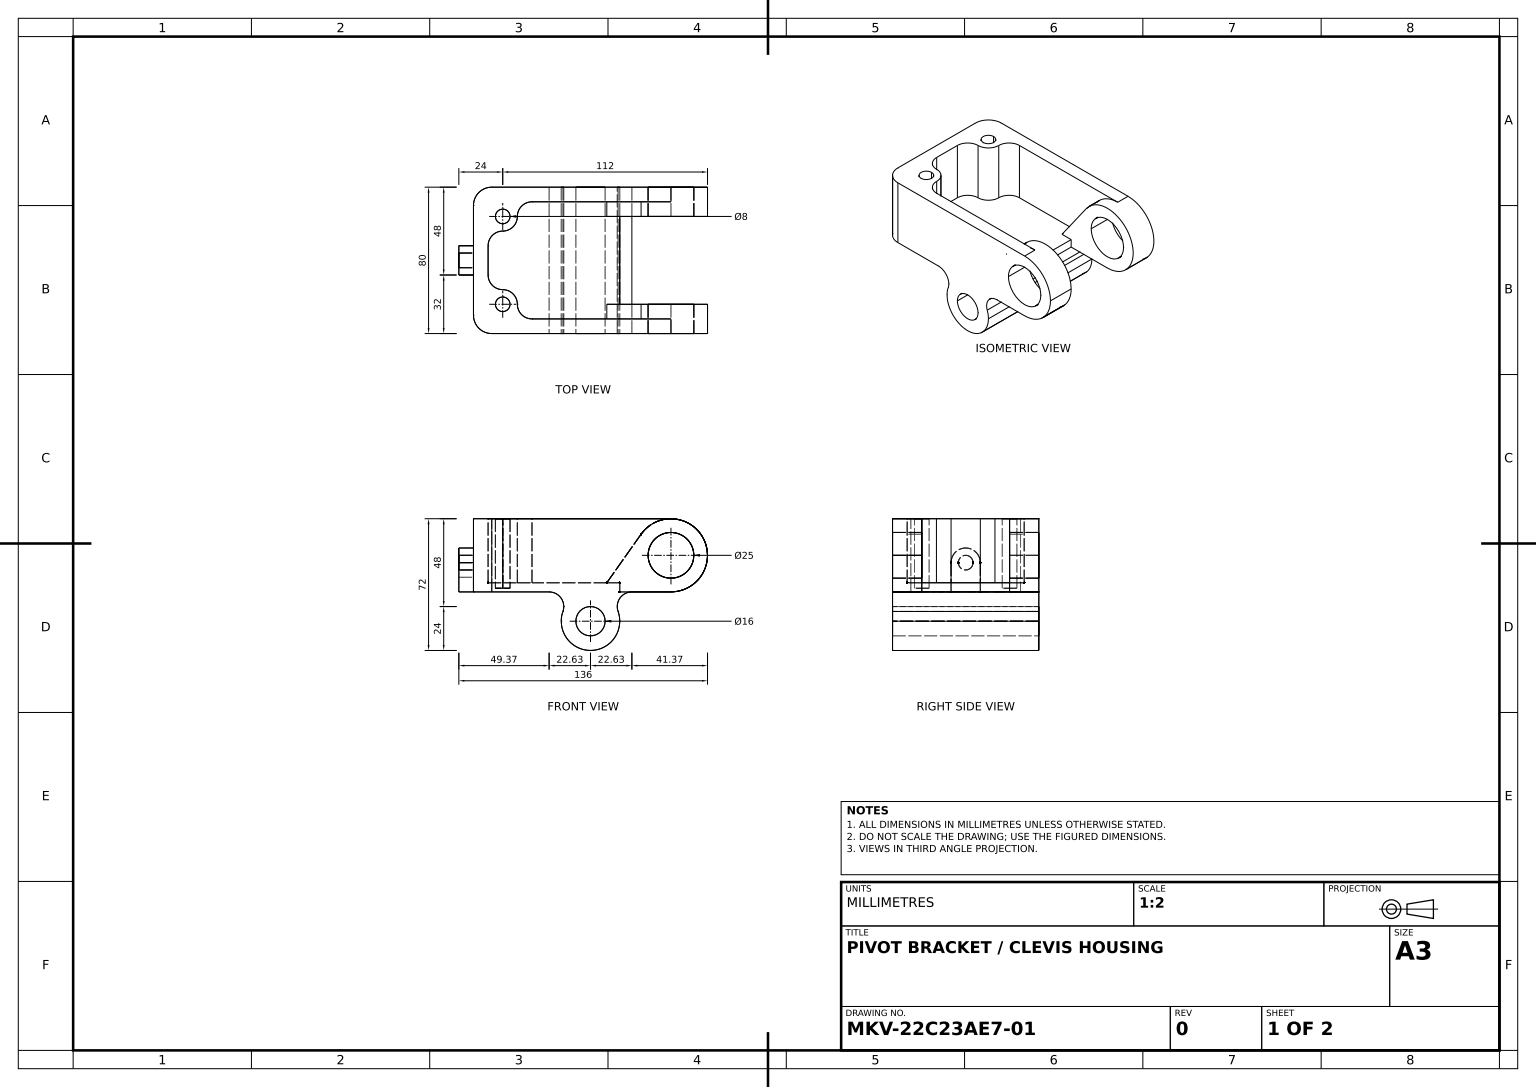
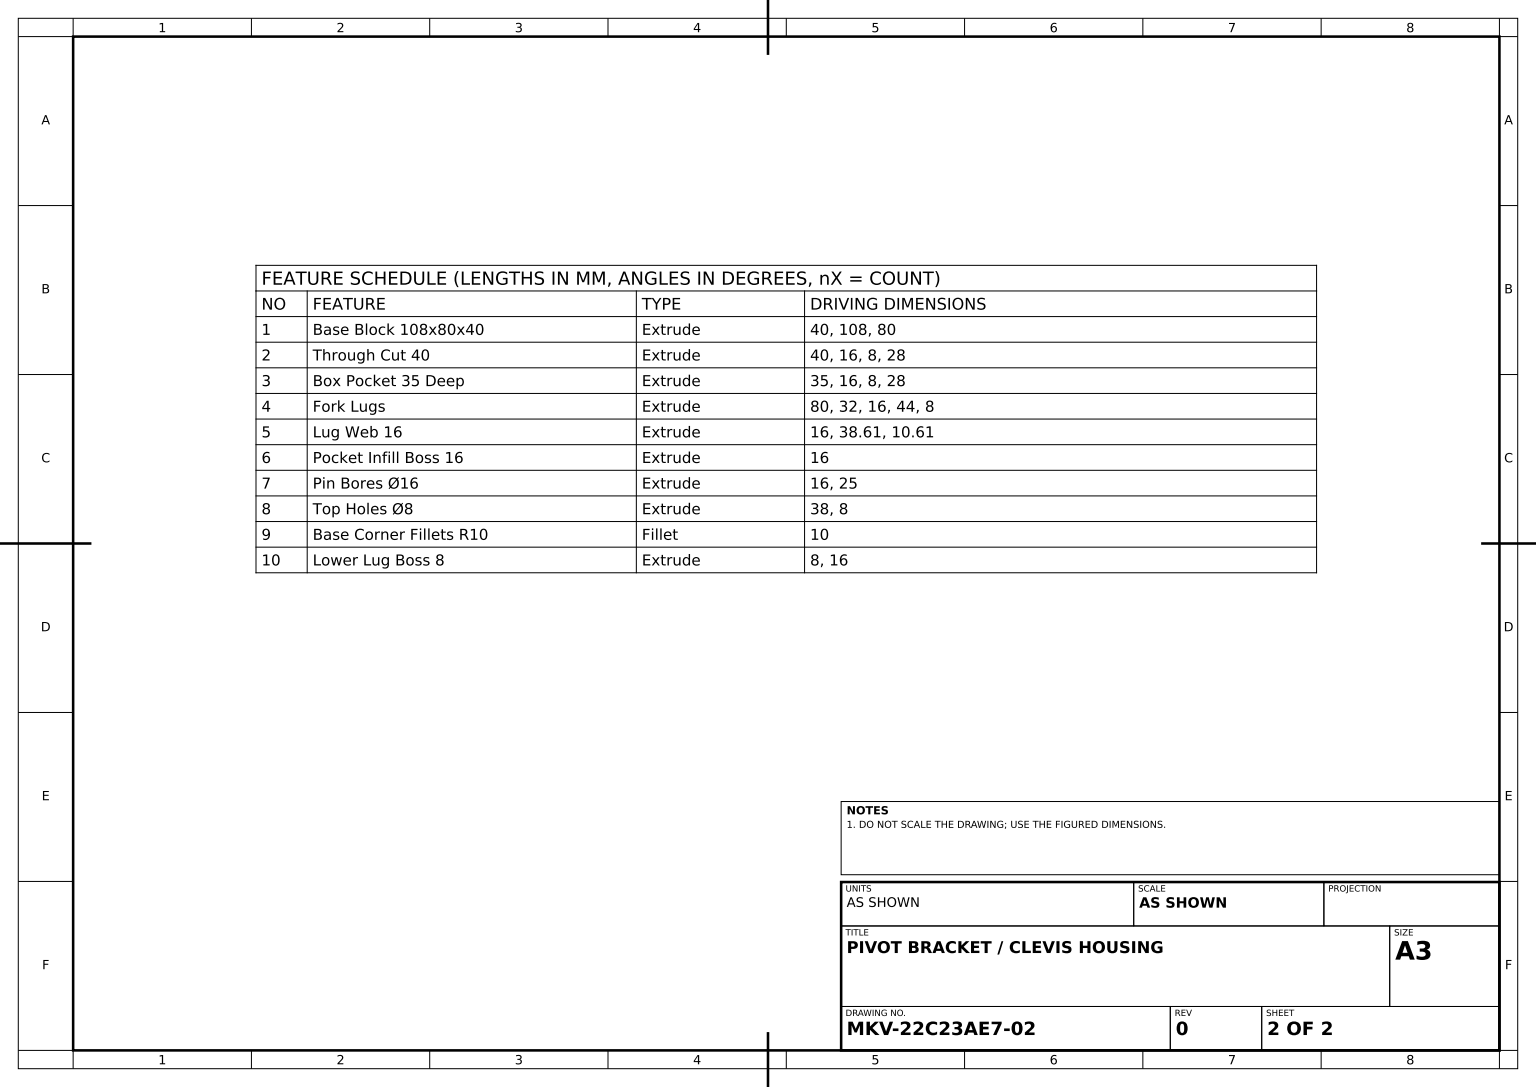
solid
v1 (-38,2,-20)
v2 (-38,40,-20)
e1 v1 v2 LINE
v3 (-38,2,-28)
e2 v3 v1 CIRCLE(AX(P(-38,2,-24),D(0,1,0),D(0,0,1)),4)
v4 (-38,40,-28)
e3 v3 v4 LINE
e4 v4 v2 CIRCLE(AX(P(-38,40,-24),D(0,1,0),D(0,0,1)),4)
face CYL(AX(P(-38,2,-24),D(0,1,0),D(0,0,1)),4) rev [-e1 -e2 e3 e4]
v5 (-38,2,28)
v6 (-38,2,20)
e5 v5 v6 CIRCLE(AX(P(-38,2,24),D(0,1,0),D(0,0,1)),4)
e6 v6 v5 CIRCLE(AX(P(-38,2,24),D(0,1,0),D(0,0,1)),4)
face PLANE(AX(P(-38,2,24),D(0,1,0),D(0,0,1))) [e5 e6]
v7 (-5.084945,-10.666667,-40)
v8 (-5.084945,-10.666667,40)
e7 v7 v8 LINE
v9 (-6,-16,-40)
e8 v7 v9 CIRCLE(AX(P(10,-16,-40),D(0,0,1),D(1,0,0)),16)
v10 (-6,-16,40)
e9 v9 v10 LINE
e10 v8 v10 CIRCLE(AX(P(10,-16,40),D(0,0,1),D(1,0,0)),16)
face CYL(AX(P(10,-16,-40),D(0,0,1),D(1,0,0)),16) [-e7 e8 e9 -e10]
v11 (74,20,24)
v12 (74,20,40)
e11 v11 v12 LINE
v13 (54,0,40)
e12 v13 v12 CIRCLE(AX(P(54,20,40),D(0,0,1),D(1,0,0)),20)
v14 (54,0,24)
e13 v13 v14 LINE
e14 v14 v11 CIRCLE(AX(P(54,20,24),D(0,0,1),D(1,0,0)),20)
face CYL(AX(P(54,20,24),D(0,0,1),D(1,0,0)),20) [e11 -e12 e13 e14]
v15 (66.5,20,24)
v16 (66.5,20,40)
e15 v15 v16 LINE
v17 (41.5,20,24)
e16 v15 v17 CIRCLE(AX(P(54,20,24),D(0,0,-1),D(-1,0,0)),12.5)
v18 (41.5,20,40)
e17 v17 v18 LINE
e18 v18 v16 CIRCLE(AX(P(54,20,40),D(0,0,1),D(1,0,0)),12.5)
face CYL(AX(P(54,20,-40),D(0,0,1),D(1,0,0)),12.5) rev [-e15 e16 e17 e18]
v19 (-30,5,24)
v20 (-38,5,16)
e19 v19 v20 CIRCLE(AX(P(-38,5,24),D(0,1,0),D(0,0,1)),8)
v21 (-38,40,16)
e20 v20 v21 LINE
v22 (-30,40,24)
e21 v22 v21 CIRCLE(AX(P(-38,40,24),D(0,1,0),D(0,0,1)),8)
e22 v19 v22 LINE
face CYL(AX(P(-38,5,24),D(0,1,0),D(0,0,1)),8) [e19 e20 -e21 -e22]
e23 v2 v4 CIRCLE(AX(P(-38,40,-24),D(0,1,0),D(0,0,1)),4)
e24 v1 v3 CIRCLE(AX(P(-38,2,-24),D(0,1,0),D(0,0,1)),4)
face CYL(AX(P(-38,2,-24),D(0,1,0),D(0,0,1)),4) rev [e23 -e3 -e24 e1]
v23 (-54,16,4)
v24 (-54,16,-4)
e25 v23 v24 CIRCLE(AX(P(-54,16,0),D(-1,0,0),D(0,0,1)),4)
v25 (-62,16,4)
e26 v25 v23 LINE
v26 (-62,16,-4)
e27 v25 v26 CIRCLE(AX(P(-62,16,0),D(-1,0,0),D(0,0,1)),4)
e28 v26 v24 LINE
face CYL(AX(P(-62,16,0),D(1,0,0),D(0,0,-1)),4) rev [-e25 -e26 e27 e28]
v27 (-22,5,-32)
v28 (-22,40,-32)
e29 v27 v28 LINE
v29 (-30,40,-24)
e30 v29 v28 CIRCLE(AX(P(-22,40,-24),D(0,-1,0),D(0,0,1)),8)
v30 (-30,5,-24)
e31 v30 v29 LINE
e32 v30 v27 CIRCLE(AX(P(-22,5,-24),D(0,-1,0),D(0,0,1)),8)
face CYL(AX(P(-22,5,-24),D(0,1,0),D(0,0,1)),8) rev [e29 -e30 -e31 e32]
e33 v24 v23 CIRCLE(AX(P(-54,16,0),D(-1,0,0),D(0,0,1)),4)
face PLANE(AX(P(-54,40,40),D(1,0,0),D(0,0,-1))) rev [e33 e25]
v31 (-44,0,40)
v32 (-54,0,30)
e34 v31 v32 CIRCLE(AX(P(-44,0,30),D(0,-1,0),D(0,0,-1)),10)
v33 (-54,0,8)
e35 v33 v32 LINE
v34 (-62,0,8)
e36 v34 v33 LINE
v35 (-62,0,-8)
e37 v35 v34 LINE
v36 (-54,0,-8)
e38 v35 v36 LINE
v37 (-54,0,-30)
e39 v37 v36 LINE
v38 (-44,0,-40)
e40 v37 v38 CIRCLE(AX(P(-44,0,-30),D(0,-1,0),D(0,0,-1)),10)
v39 (-12.627417,0,-40)
e41 v39 v38 LINE
v40 (-12.627417,0,40)
e42 v39 v40 LINE
e43 v31 v40 LINE
face PLANE(AX(P(0,0,0),D(0,-1,0),D(0,0,-1))) [e34 -e35 -e36 -e37 e38 -e39 e40 -e41 e42 -e43]
v41 (66.5,20,-40)
v42 (66.5,20,-24)
e44 v41 v42 LINE
v43 (41.5,20,-24)
e45 v43 v42 CIRCLE(AX(P(54,20,-24),D(0,0,-1),D(-1,0,0)),12.5)
v44 (41.5,20,-40)
e46 v44 v43 LINE
e47 v41 v44 CIRCLE(AX(P(54,20,-40),D(0,0,1),D(1,0,0)),12.5)
face CYL(AX(P(54,20,-40),D(0,0,1),D(1,0,0)),12.5) rev [e44 -e45 -e46 -e47]
v45 (-62,16,-8)
v46 (-54,16,-8)
e48 v45 v46 LINE
v47 (-62,16,8)
e49 v47 v45 CIRCLE(AX(P(-62,16,0),D(-1,0,0),D(0,0,1)),8)
v48 (-54,16,8)
e50 v47 v48 LINE
e51 v48 v46 CIRCLE(AX(P(-54,16,0),D(-1,0,0),D(0,0,1)),8)
face CYL(AX(P(-62,16,0),D(1,0,0),D(0,0,-1)),8) [-e48 -e49 e50 e51]
v49 (2,-16,-40)
v50 (18,-16,-40)
e52 v49 v50 CIRCLE(AX(P(10,-16,-40),D(0,0,1),D(1,0,0)),8)
e53 v50 v49 CIRCLE(AX(P(10,-16,-40),D(0,0,1),D(1,0,0)),8)
e54 v44 v41 CIRCLE(AX(P(54,20,-40),D(0,0,1),D(1,0,0)),12.5)
v51 (-4.627417,-8,-40)
e55 v51 v7 CIRCLE(AX(P(-12.627417,-8,-40),D(0,0,-1),D(-1,0,0)),8)
e56 v39 v51 CIRCLE(AX(P(-12.627417,-8,-40),D(0,0,-1),D(-1,0,0)),8)
v52 (-44,40,-40)
e57 v38 v52 LINE
v53 (54,40,-40)
e58 v53 v52 LINE
v54 (54,0,-40)
e59 v53 v54 CIRCLE(AX(P(54,20,-40),D(0,0,-1),D(-1,0,0)),20)
v55 (32.627417,0,-40)
e60 v54 v55 LINE
v56 (25.084945,-10.666667,-40)
e61 v56 v55 CIRCLE(AX(P(32.627417,-8,-40),D(0,0,-1),D(-1,0,0)),8)
v57 (26,-16,-40)
e62 v57 v56 CIRCLE(AX(P(10,-16,-40),D(0,0,1),D(1,0,0)),16)
e63 v9 v57 CIRCLE(AX(P(10,-16,-40),D(0,0,1),D(1,0,0)),16)
face PLANE(AX(P(-54,40,-40),D(0,0,1),D(1,0,0))) rev [e52 e53] [e54 e47] [-e8 -e55 -e56 e41 e57 -e58 e59 e60 -e61 -e62 -e63]
v58 (26,5,24)
v59 (18.921249,5,24)
e64 v58 v59 LINE
v60 (37.663471,31.537669,24)
e65 v60 v59 LINE
e66 v11 v60 CIRCLE(AX(P(54,20,24),D(0,0,1),D(1,0,0)),20)
v61 (32.627417,0,24)
e67 v61 v14 LINE
v62 (26,0,24)
e68 v61 v62 LINE
e69 v58 v62 LINE
e70 v17 v15 CIRCLE(AX(P(54,20,24),D(0,0,-1),D(-1,0,0)),12.5)
face PLANE(AX(P(32.627417,-8,24),D(0,0,-1),D(-1,0,0))) [e64 -e65 -e66 -e14 -e67 e68 -e69] [-e70 -e16]
v63 (32.627417,0,-24)
e71 v55 v63 LINE
e72 v63 v61 LINE
v64 (32.627417,0,40)
e73 v61 v64 LINE
v65 (25.084945,-10.666667,40)
e74 v65 v64 CIRCLE(AX(P(32.627417,-8,40),D(0,0,-1),D(-1,0,0)),8)
e75 v56 v65 LINE
face CYL(AX(P(32.627417,-8,-40),D(0,0,1),D(1,0,0)),8) rev [e61 e71 e72 e73 -e74 -e75]
v66 (18,-16,40)
e76 v50 v66 LINE
v67 (2,-16,40)
e77 v66 v67 CIRCLE(AX(P(10,-16,40),D(0,0,1),D(1,0,0)),8)
e78 v49 v67 LINE
face CYL(AX(P(10,-16,-40),D(0,0,1),D(1,0,0)),8) rev [e76 e77 -e78 -e53]
v68 (-54,40,-30)
e79 v52 v68 CIRCLE(AX(P(-44,40,-30),D(0,1,0),D(0,0,-1)),10)
v69 (-54,40,30)
e80 v68 v69 LINE
v70 (-44,40,40)
e81 v69 v70 CIRCLE(AX(P(-44,40,30),D(0,1,0),D(0,0,-1)),10)
v71 (54,40,40)
e82 v70 v71 LINE
v72 (54,40,32)
e83 v71 v72 LINE
v73 (-22,40,32)
e84 v72 v73 LINE
e85 v22 v73 CIRCLE(AX(P(-22,40,24),D(0,1,0),D(0,0,1)),8)
v74 (-46,40,8)
e86 v74 v21 CIRCLE(AX(P(-38,40,8),D(0,1,0),D(0,0,1)),8)
v75 (-46,40,-8)
e87 v74 v75 LINE
v76 (-38,40,-16)
e88 v75 v76 CIRCLE(AX(P(-38,40,-8),D(0,-1,0),D(0,0,1)),8)
e89 v76 v29 CIRCLE(AX(P(-38,40,-24),D(0,1,0),D(0,0,1)),8)
v77 (54,40,-32)
e90 v77 v28 LINE
e91 v77 v53 LINE
v78 (-38,40,20)
v79 (-38,40,28)
e92 v78 v79 CIRCLE(AX(P(-38,40,24),D(0,1,0),D(0,0,1)),4)
e93 v79 v78 CIRCLE(AX(P(-38,40,24),D(0,1,0),D(0,0,1)),4)
face PLANE(AX(P(0,40,0),D(0,-1,0),D(0,0,-1))) rev [e79 e80 e81 e82 e83 e84 -e85 e21 -e86 e87 e88 e89 e30 -e90 e91 e58] [-e4 -e23] [-e92 -e93]
e94 v64 v13 LINE
face PLANE(AX(P(0,0,0),D(0,-1,0),D(0,0,-1))) [e67 -e13 -e94 -e73]
v80 (-22,5,32)
e95 v19 v80 CIRCLE(AX(P(-22,5,24),D(0,1,0),D(0,0,1)),8)
v81 (18.921249,5,32)
e96 v81 v80 LINE
e97 v59 v81 LINE
v82 (26,5,-24)
e98 v82 v58 LINE
v83 (18.921249,5,-24)
e99 v82 v83 LINE
v84 (18.921249,5,-32)
e100 v83 v84 LINE
e101 v84 v27 LINE
v85 (-38,5,-16)
e102 v85 v30 CIRCLE(AX(P(-38,5,-24),D(0,1,0),D(0,0,1)),8)
v86 (-46,5,-8)
e103 v86 v85 CIRCLE(AX(P(-38,5,-8),D(0,-1,0),D(0,0,1)),8)
v87 (-46,5,8)
e104 v87 v86 LINE
e105 v87 v20 CIRCLE(AX(P(-38,5,8),D(0,1,0),D(0,0,1)),8)
face PLANE(AX(P(0,5,0),D(0,1,0),D(0,0,1))) [e95 -e96 -e97 -e64 -e98 e99 e100 e101 -e32 -e102 -e103 -e104 e105 -e19]
e106 v32 v69 LINE
e107 v68 v37 LINE
e108 v46 v36 LINE
e109 v33 v48 LINE
face PLANE(AX(P(-54,40,40),D(1,0,0),D(0,0,-1))) rev [e106 -e80 e107 e39 -e108 -e51 -e109 e35]
e110 v85 v76 LINE
face CYL(AX(P(-38,5,-24),D(0,1,0),D(0,0,1)),8) [-e89 -e110 e102 e31]
v88 (37.663471,31.537669,-24)
e111 v83 v88 LINE
v89 (37.663471,31.537669,-32)
e112 v88 v89 LINE
e113 v84 v89 LINE
face PLANE(AX(P(18.921249,5,-24),D(-0.816826456,0.576883473,0),D(-0.576883473,-0.816826456,0))) [e111 e112 -e113 -e100]
v90 (37.663471,31.537669,32)
e114 v90 v72 CIRCLE(AX(P(54,20,32),D(0,0,-1),D(-1,0,0)),20)
e115 v81 v90 LINE
e116 v80 v73 LINE
face PLANE(AX(P(0,0,32),D(0,0,-1),D(-1,0,0))) [-e114 -e115 e96 e116 -e84]
v91 (26,-16,40)
e117 v57 v91 LINE
e118 v10 v91 CIRCLE(AX(P(10,-16,40),D(0,0,1),D(1,0,0)),16)
face CYL(AX(P(10,-16,-40),D(0,0,1),D(1,0,0)),16) [e117 -e118 -e9 e63]
e119 v67 v66 CIRCLE(AX(P(10,-16,40),D(0,0,1),D(1,0,0)),8)
face CYL(AX(P(10,-16,-40),D(0,0,1),D(1,0,0)),8) rev [e119 -e76 -e52 e78]
e120 v5 v79 LINE
e121 v6 v78 LINE
face CYL(AX(P(-38,2,24),D(0,1,0),D(0,0,1)),4) rev [-e5 e120 e93 -e121]
e122 v34 v47 LINE
e123 v45 v35 LINE
e124 v26 v25 CIRCLE(AX(P(-62,16,0),D(-1,0,0),D(0,0,1)),4)
face PLANE(AX(P(-62,16,0),D(-1,0,0),D(0,0,1))) [e37 e122 e49 e123] [-e27 -e124]
face CYL(AX(P(-22,5,24),D(0,1,0),D(0,0,1)),8) rev [-e95 e22 e85 -e116]
e125 v86 v75 LINE
face CYL(AX(P(-38,5,-8),D(0,1,0),D(0,0,1)),8) rev [-e125 e103 e110 -e88]
face CYL(AX(P(-38,2,24),D(0,1,0),D(0,0,1)),4) rev [e121 e92 -e120 -e6]
e126 v91 v65 CIRCLE(AX(P(10,-16,40),D(0,0,1),D(1,0,0)),16)
face CYL(AX(P(10,-16,-40),D(0,0,1),D(1,0,0)),16) [e62 e75 -e126 -e117]
v92 (-4.627417,-8,40)
e127 v92 v8 CIRCLE(AX(P(-12.627417,-8,40),D(0,0,-1),D(-1,0,0)),8)
e128 v12 v71 CIRCLE(AX(P(54,20,40),D(0,0,1),D(1,0,0)),20)
e129 v70 v31 LINE
e130 v40 v92 CIRCLE(AX(P(-12.627417,-8,40),D(0,0,-1),D(-1,0,0)),8)
e131 v16 v18 CIRCLE(AX(P(54,20,40),D(0,0,1),D(1,0,0)),12.5)
face PLANE(AX(P(-54,40,40),D(0,0,-1),D(-1,0,0))) rev [-e77 -e119] [e127 e10 e118 e126 e74 e94 e12 e128 -e82 e129 e43 e130] [-e131 -e18]
face PLANE(AX(P(-62,16,-8),D(0,0,1),D(1,0,0))) rev [-e123 e48 e108 -e38]
face CYL(AX(P(54,20,-40),D(0,0,1),D(1,0,0)),12.5) rev [e15 e131 -e17 e70]
e132 v51 v92 LINE
face CYL(AX(P(-12.627417,-8,-40),D(0,0,1),D(1,0,0)),8) rev [-e42 e56 e132 -e130]
face CYL(AX(P(-44,40,30),D(0,-1,0),D(0,0,-1)),10) [-e106 -e34 -e129 -e81]
e133 v42 v43 CIRCLE(AX(P(54,20,-24),D(0,0,-1),D(-1,0,0)),12.5)
v93 (54,0,-24)
e134 v88 v93 CIRCLE(AX(P(54,20,-24),D(0,0,-1),D(-1,0,0)),20)
v94 (26,0,-24)
e135 v94 v82 LINE
e136 v63 v94 LINE
e137 v93 v63 LINE
face PLANE(AX(P(32.627417,-8,-24),D(0,0,-1),D(-1,0,0))) rev [e45 e133] [-e134 -e111 -e99 -e135 -e136 -e137]
e138 v93 v54 LINE
face PLANE(AX(P(0,0,0),D(0,-1,0),D(0,0,-1))) [-e60 -e138 e137 -e71]
e139 v89 v77 CIRCLE(AX(P(54,20,-32),D(0,0,-1),D(-1,0,0)),20)
face PLANE(AX(P(0,0,-32),D(0,0,-1),D(-1,0,0))) rev [e113 e139 e90 -e29 -e101]
e140 v60 v90 LINE
face CYL(AX(P(54,20,24),D(0,0,1),D(1,0,0)),20) [e114 -e83 -e128 -e11 e66 e140]
face PLANE(AX(P(37.663471,31.537669,24),D(-0.816826456,0.576883473,0),D(-0.576883473,-0.816826456,0))) [e97 e115 -e140 e65]
e141 v94 v62 LINE
face PLANE(AX(P(26,0,0),D(-1,0,0),D(0,0,1))) rev [e69 -e141 e135 e98]
face CYL(AX(P(-44,40,-30),D(0,-1,0),D(0,0,-1)),10) [-e79 -e57 -e40 -e107]
face PLANE(AX(P(-62,0,8),D(0,0,-1),D(-1,0,0))) rev [-e50 -e122 e36 e109]
e142 v87 v74 LINE
face CYL(AX(P(-38,5,8),D(0,1,0),D(0,0,1)),8) rev [e86 -e20 -e105 e142]
face PLANE(AX(P(-12.627417,0,-40),D(0,1,0),D(0,0,1))) [-e68 -e72 e136 e141]
face PLANE(AX(P(-38,2,-24),D(0,1,0),D(0,0,1))) [e24 e2]
face CYL(AX(P(-62,16,0),D(1,0,0),D(0,0,-1)),4) rev [e26 -e33 -e28 e124]
face PLANE(AX(P(-46,5,0),D(1,0,0),D(0,0,-1))) [e125 -e87 -e142 e104]
face CYL(AX(P(54,20,-40),D(0,0,1),D(1,0,0)),12.5) rev [e46 -e133 -e44 -e54]
face CYL(AX(P(-12.627417,-8,-40),D(0,0,1),D(1,0,0)),8) rev [e55 e7 -e127 -e132]
face CYL(AX(P(54,20,-24),D(0,0,-1),D(-1,0,0)),20) [-e91 -e139 -e112 e134 e138 -e59]
